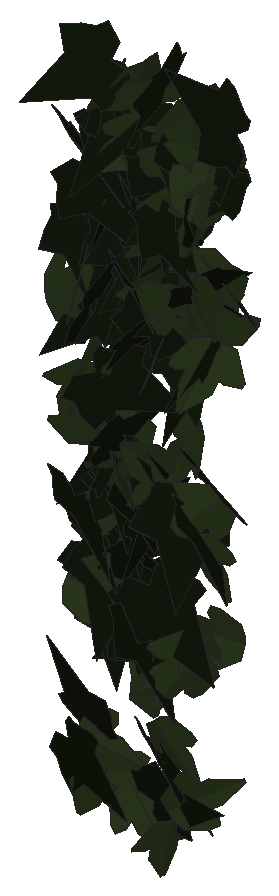
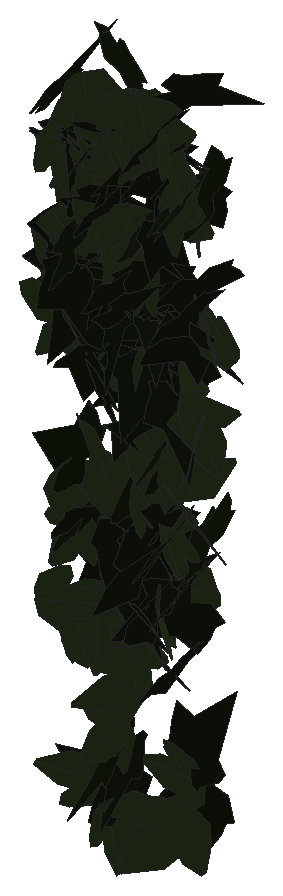
# SketchUp Ruby script. Lengths in inches.
U = 1.inch
M = Sketchup.active_model
def pt(a) = Geom::Point3d.new(a.map { |v| v * U })
def face(e, loops, mat)
  f = e.add_face(loops[0].map { |a| pt(a) })
  loops[1..].each { |l| e.add_face(l.map { |a| pt(a) }).erase! }
  f.material = f.back_material = mat if mat
  f
end
# faces: each face lists its corners as indices into pts; further lists are holes
def faces(e, pts, list, mat = nil) = list.each { |f| face(e, (f[0].is_a?(Array) ? f : [f]).map { |l| l.map { |i| pts[i] } }, mat) }
# xy, xz, yz: faces in a plane at the given z, y or x. An outline is a flat list of corners, or four numbers for a rectangle; further outlines are holes
def ring(l) = l.size == 4 ? [[l[0], l[1]], [l[2], l[1]], [l[2], l[3]], [l[0], l[3]]] : l.each_slice(2).to_a
def flat(e, list, mat, &to3) = list.each { |f| face(e, (f[0].is_a?(Array) ? f : [f]).map { |l| ring(l).map { |u, v| to3.(u, v) } }, mat) }
def xy(e, z, list, mat = nil) = flat(e, list, mat) { |x, y| [x, y, z] }
def xz(e, y, list, mat = nil) = flat(e, list, mat) { |x, z| [x, y, z] }
def yz(e, x, list, mat = nil) = flat(e, list, mat) { |y, z| [x, y, z] }
def lines(e, pts, list) = list.each { |a, b| e.add_line(pt(pts[a]), pt(pts[b])) }
# prism: a flat outline (further loops are holes) pulled along v
def prism(e, loops, v, mat = nil)
  f = face(e, loops, mat); d = Geom::Vector3d.new(v.map { |x| x * U })
  f.pushpull(f.normal.samedirection?(d) ? d.length : -d.length)
end
def box(e, o, s, mat = nil) = prism(e, [[o, [o[0] + s[0], o[1], o[2]], [o[0] + s[0], o[1] + s[1], o[2]], [o[0], o[1] + s[1], o[2]]]], [0, 0, s[2]], mat)
def at(x, y, z, deg = 0) = Geom::Transformation.translation(pt([x, y, z])) * Geom::Transformation.rotation(ORIGIN, Z_AXIS, deg.degrees)
def axes(o, x, y, z) = Geom::Transformation.new([*x, 0, *y, 0, *z, 0, *pt(o).to_a, 1])
def part(name) = M.definitions.add(name)
# library, detail: a bought-in or finely detailed component or shape, given as its bounding box
def library(name, o, s) = part(name).tap { |d| box(d.entities, o, s) }
def detail(e, o, s) = box(e.add_group.entities, o, s)
def put(e, d, t, mat = nil) = e.add_instance(d, t).tap { |i| i.material = mat if mat }
def group(e, t, mat = nil) = e.add_group.tap { |g| g.transformation = t; g.material = mat if mat }.entities
root = M.entities
M.materials.add("efeu1").color = [18, 25, 13]
M.materials.add("efeu2").color = [43, 57, 29]
c1 = part("ivyleaf_10")
p = [[0,0.5,-0.03],[-0.0625,2.02,-0.43],[-0.19,2.01,-0.46],[-0.54,1.05,-0.29],[-0.52,0.625,-0.18],[-0.83,0.76,-0.28],
  [-1.16,0.64,-0.33],[-1.15,0.33,-0.24],[-0.77,-0.39,0.02],[-0.3,-0.51,0.16],[0.04,-0.48,0.23],[-0.02,2.01,-0.4375],
  [-0.06,2.01,-0.43],[0.04,-0.49,0.23],[0.67,-0.49,0.14],[1.38,0.36,-0.2],[1.375,0.51,-0.24],[0.81,0.65,-0.19],
  [0.62,0.59,-0.15],[0.6,1.09,-0.28],[0.5,1.23,-0.31]]
faces(c1.entities,p,[[0,1,2,3,4,5,6,7,8,9,10],[11,12,0,13,14,15,16,17,18,19,20]],"efeu2")
c2 = part("ivyleaf_9")
p = [[1.54,2.16,1.25],[1.36,2.04,1.19],[-0.21,0.99,0.68],[-0.71,1.11,0.82],[-0.85,0.86,0.67],[-0.8,0.17,0.21],
  [-0.9,-0.01,0.1],[-0.67,-0.16,-0.02],[-0.08,-0.08,-0.05],[-0.03,-0.6,-0.4],[0.65,-0.88,-0.66],[0.83,-0.6,-0.49],
  [1.29,-0.42,-0.43],[1.8125,-0.07,-0.26],[1.21,0.44,0.15]]
faces(c2.entities,p,[[0,1,2,3,4,5,6,7,8,9,10,11,12,13,14]],"efeu1")
put(root,c1,axes([538.125,133.94,196.47],[-0.39679,-0.64724,0.32465],[-0.18478,-0.26744,-0.75901],[0.70012,-0.4374,-0.01633]))
put(root,c1,axes([538.48,134.31,202.8],[0.11635,0.17729,-0.84393],[-0.75483,0.43271,-0.01316],[0.41698,0.73384,0.21165]))
put(root,c1,axes([537.35,133.61,198.76],[0.54882,-0.22672,-0.62542],[0.56928,-0.25944,0.59361],[-0.3442,-0.7906,-0.01544]))
put(root,c2,axes([537.7,135.02,200.15],[-0.06376,-0.80231,0.12393],[-0.00926,-0.12358,-0.80484],[0.81178,-0.06443,0.00055]))
put(root,c1,axes([537.86,133.92,199.76],[0.55544,-0.65414,0.12328],[0.08516,-0.08941,-0.85812],[0.66019,0.56189,0.00697]))
put(root,c2,axes([537.78,134.2,200.82],[-0.09395,-0.79589,-0.21894],[0.03485,0.21634,-0.80136],[0.82472,-0.0998,0.00892]))
put(root,c2,axes([537.42,134.14,203.42],[0.58741,-0.58266,0.31966],[0.22728,-0.22478,-0.82737],[0.62451,0.62984,0.00043]))
put(root,c2,axes([538.35,133.75,186.3125],[0.41543,-0.40758,0.66623],[-0.47527,0.46689,0.58198],[-0.61976,-0.63124,0.00028]))
put(root,c1,axes([538.19,133.99,203.29],[0.50827,-0.5984,-0.32039],[-0.1439,0.29617,-0.78144],[0.66334,0.52275,0.07598]))
put(root,c1,axes([538.22,133.96,195.16],[-0.37011,0.76913,-0.02259],[-0.02989,0.01068,0.85325],[0.76888,0.37064,0.02229]))
put(root,c1,axes([538.09,134.36,197.58],[-0.22239,0.34672,-0.67417],[-0.01153,-0.70404,-0.35828],[-0.75801,-0.09102,0.20324]))
put(root,c2,axes([537.76,134.75,203.42],[0.47419,-0.67063,-0.05659],[0.01118,0.07706,-0.8196],[0.67292,0.4713,0.05349]))
put(root,c1,axes([538.29,134.74,204.97],[0.18494,-0.82253,0.03934],[0.01737,-0.03641,-0.84302],[0.82329,0.18553,0.00895]))
put(root,c2,axes([538.625,134.12,194.17],[-0.70422,0.30749,-0.05921],[0.05562,-0.02059,-0.76841],[-0.30816,-0.7064,-0.00337]))
put(root,c2,axes([538.68,133.97,205.98],[-0.66134,-0.30761,0.44171],[-0.35877,-0.26973,-0.72501],[0.40127,-0.74815,0.07978]))
put(root,c1,axes([538.23,134.01,194.68],[-0.74503,-0.50115,0.12123],[0.10127,0.06665,0.8979],[-0.50556,0.75188,0.00122]))
put(root,c2,axes([537.8,133.77,192.81],[0.42266,-0.77344,0.38973],[0.22896,-0.31845,-0.88029],[0.83527,0.47867,0.04409]))
put(root,c2,axes([538.81,133.8125,199.04],[-0.83451,0.00371,0.04795],[-0.04795,0.00106,-0.83451],[-0.00377,-0.83588,-0.00085]))
put(root,c2,axes([538.13,134.6875,191.55],[0.06127,-0.74917,0.31351],[0.01739,-0.31312,-0.75163],[0.81193,0.06324,-0.00756]))
put(root,c2,axes([538.75,133.83,196.84],[-0.1433,0.76912,-0.04322],[0.00941,-0.04221,-0.78235],[-0.77028,-0.1436,-0.00152]))
put(root,c2,axes([538.65,133.17,198.97],[-0.20834,0.44217,-0.79802],[-0.44743,0.66384,0.48464],[0.79508,0.48944,0.06362]))
put(root,c2,axes([537.89,133.46,185.6],[-0.00066,0.00453,-0.90717],[0.85758,0.29587,0.00085],[0.29587,-0.85757,-0.0045]))
put(root,c2,axes([538.29,134.65,189.38],[0.10566,-0.80781,0.08287],[0.01503,-0.08161,-0.81468],[0.81191,0.10663,0.0043]))
put(root,c2,axes([538.1,134.2,191.24],[0.03261,-0.15185,-0.83319],[0.40483,0.73517,-0.11815],[0.74389,-0.39343,0.10081]))
put(root,c1,axes([538.59,134.36,193.08],[0.75086,-0.1518,-0.07309],[-0.0714,0.01567,-0.76605],[0.1526,0.75425,0.0012]))
put(root,c2,axes([538.31,135.02,193.11],[0.16744,-0.77195,0.31509],[0.09835,-0.30085,-0.78933],[0.82796,0.19185,0.03004]))
put(root,c2,axes([538.17,133.66,192.39],[0.43223,-0.67212,0.32669],[0.17237,-0.27755,-0.79909],[0.72715,0.46531,-0.00477]))
put(root,c2,axes([538.82,134.6,202.29],[-0.39025,0.41969,-0.60601],[0.40578,-0.45015,-0.57306],[-0.61541,-0.56295,0.00644]))
put(root,c1,axes([538.52,134.7,191.02],[0.42529,-0.56538,0.53829],[0.36777,-0.39559,-0.70607],[0.68859,0.56048,0.04465]))
put(root,c1,axes([538.41,134.07,184.56],[-0.56636,-0.35628,-0.73053],[0.63915,0.35482,-0.66856],[0.5021,-0.85355,0.02701]))
put(root,c2,axes([538.65,134.82,204.08],[0.03151,-0.83531,-0.00958],[0.00016,0.00959,-0.8359],[0.83537,0.0315,0.00052]))
put(root,c1,axes([539.18,133.84,193.42],[-0.85254,0.32496,-0.16501],[-0.16092,0.041,0.91218],[0.327,0.86739,0.0187]))
put(root,c1,axes([539.34,134.13,195.35],[-0.4903,-0.3673,0.47625],[-0.29142,-0.39241,-0.60266],[0.52611,-0.55966,0.11001]))
put(root,c2,axes([538.74,134.9375,204.88],[0.08119,-0.8197,0.15461],[-0.00481,-0.15579,-0.82348],[0.83414,0.07889,-0.0198]))
put(root,c1,axes([538.4,133.77,185.78],[-0.09107,-0.04313,-0.87343],[0.82011,-0.30906,-0.07025],[-0.30358,-0.82198,0.07224]))
put(root,c2,axes([538.75,134.41,193.63],[0.08448,-0.46343,-0.66386],[0.03174,0.66885,-0.46288],[0.80899,0.02216,0.08749]))
put(root,c2,axes([539.19,134,204.42],[-0.77309,-0.18213,-0.23459],[0.27024,-0.16004,-0.76631],[0.12319,-0.79189,0.20882]))
put(root,c1,axes([539.18,134.7,205.51],[-0.09843,-0.84393,-0.00061],[0.00258,0.00031,-0.84964],[0.84392,-0.09843,0.00252]))
put(root,c2,axes([538.72,133.39,202.96],[-0.21372,-0.39699,-0.75706],[0.36359,0.66404,-0.45085],[0.77365,-0.42174,0.00275]))
put(root,c1,axes([539.08,134.82,194.43],[0.13144,-0.711,0.4615],[0.16516,-0.43658,-0.71965],[0.8314,0.19914,0.07]))
put(root,c2,axes([538.74,135.12,202.21],[0.10311,-0.68691,0.42719],[0.20691,-0.39393,-0.68336],[0.78201,0.1948,0.12448]))
put(root,c2,axes([538.92,134.51,200.82],[-0.30169,-0.59253,-0.4913],[0.24506,0.42629,-0.66461],[0.72967,-0.38816,0.02008]))
put(root,c2,axes([538.78,134.47,195.58],[0.41385,-0.68545,0.07201],[0.05112,-0.05324,-0.80053],[0.68732,0.41668,0.01618]))
put(root,c2,axes([538.95,133.87,191.16],[-0.03343,-0.93443,0.2435],[-0.0278,-0.24261,-0.93485],[0.96524,-0.03935,-0.01849]))
put(root,c1,axes([538.73,132.88,190.87],[0.15765,0.17631,0.79245],[0.5788,0.54163,-0.23565],[-0.56925,0.59955,-0.02015]))
put(root,c2,axes([539.74,133.74,198.74],[-0.15746,0.63778,0.51889],[-0.17108,0.49135,-0.65583],[-0.8042,-0.2294,0.03792]))
put(root,c2,axes([539.39,134.75,190.82],[-0.68632,0.01807,-0.40688],[0.40667,-0.01322,-0.68656],[-0.02229,-0.79775,0.00216]))
put(root,c2,axes([538.68,134.85,190.97],[0.33065,-0.32867,0.68533],[0.52789,-0.43841,-0.46494],[0.54685,0.62194,0.03443]))
put(root,c1,axes([539.74,134.18,204.11],[0.3884,0.38225,-0.66317],[-0.58372,-0.33316,-0.5339],[-0.49516,0.69257,0.10919]))
put(root,c2,axes([539.63,135.22,199.79],[-0.48758,-0.49086,0.40875],[-0.20865,-0.36362,-0.68556],[0.60372,-0.5221,0.09317]))
put(root,c2,axes([539.26,133.14,195.12],[0.04861,0.6858,-0.38367],[-0.05895,0.3865,0.6834],[0.78361,-0.01347,0.07521]))
put(root,c2,axes([539.47,133.83,192.05],[-0.06765,0.11804,-0.82061],[-0.25856,0.77927,0.13341],[0.7877,0.26592,-0.02669]))
put(root,c1,axes([539.43,134.4,200.57],[-0.73866,0.29447,-0.24979],[0.22395,-0.11254,-0.79493],[-0.31457,-0.77159,0.02061]))
put(root,c2,axes([539.7,133.91,197.63],[0.1711,0.75323,0.1979],[0.04561,0.19258,-0.77241],[-0.77745,0.17707,-0.00175]))
put(root,c1,axes([539.68,133.83,197.64],[0.01621,-0.75073,0.26481],[0.05305,-0.26326,-0.74957],[0.79429,0.0329,0.04466]))
put(root,c1,axes([539.75,134.35,205.33],[-0.53255,-0.62878,-0.11069],[0.05267,0.10039,-0.82363],[0.63627,-0.53459,-0.02447]))
put(root,c2,axes([539.45,134.22,192.77],[0.64452,-0.55319,-0.25391],[0.19238,-0.16572,0.84937],[-0.57748,-0.67262,-0.00044]))
put(root,c1,axes([539.66,134.5,189.28],[0.52893,0.56042,-0.0564],[-0.03982,-0.03997,-0.77061],[-0.56185,0.53043,0.00153]))
put(root,c2,axes([539.38,132.79,197.42],[0.08838,-0.02853,-0.91244],[0.18508,0.89822,-0.01016],[0.89392,-0.18315,0.09231]))
put(root,c2,axes([540.35,133.875,189.58],[-0.68311,0.31373,0.19461],[-0.18307,0.06757,-0.75157],[-0.3206,-0.70707,0.01452]))
put(root,c2,axes([540.19,134.92,199.65],[-0.29134,-0.85831,-0.02374],[0.02449,-0.03337,0.90577],[-0.85829,0.29039,0.03391]))
put(root,c1,axes([539.87,134.37,201.9],[-0.30237,-0.66513,-0.40057],[0.17699,0.35951,-0.73055],[0.756,-0.35019,0.01082]))
put(root,c2,axes([539.3,134.66,194.21],[0.65805,-0.06727,-0.51152],[0.50623,-0.07573,0.66121],[-0.09952,-0.83003,-0.01888]))
put(root,c1,axes([540.23,134.7,193.93],[-0.38247,-0.4744,-0.72554],[-0.44713,-0.57142,0.60934],[-0.74265,0.58836,0.00679]))
put(root,c2,axes([540.06,134.72,193.16],[-0.34013,0.42247,-0.77528],[0.47469,-0.61303,-0.54231],[-0.74445,-0.58391,0.00842]))
put(root,c1,axes([539.77,133.85,184.52],[0.40929,0.63903,0.34305],[0.18398,0.28954,-0.75886],[-0.70156,0.44873,0.00112]))
put(root,c2,axes([540.37,133.5,198.86],[-0.31113,0.5612,-0.46962],[0.10165,-0.47222,-0.63165],[-0.72468,-0.30718,0.11302]))
put(root,c2,axes([539.77,133.71,199.41],[-0.20769,-0.1469,0.7938],[0.31409,-0.76977,-0.06027],[0.74367,0.28409,0.24715]))
put(root,c2,axes([540.44,134.26,200.13],[-0.77869,-0.3229,0.02286],[-0.01891,-0.01406,-0.84297],[0.32316,-0.7789,0.00574]))
put(root,c2,axes([540.4375,134.2,199.34],[0.49129,0.07557,-0.68058],[-0.68457,0.07407,-0.48594],[0.01624,0.8361,0.10457]))
put(root,c2,axes([539.91,134.34,203.52],[0.32212,-0.68183,-0.35126],[-0.0747,0.35128,-0.75038],[0.76335,0.3221,0.07479]))
put(root,c2,axes([540.25,133.82,186.27],[0.70306,-0.07472,-0.51763],[-0.51061,0.08956,-0.70646],[0.11314,0.86846,0.02832]))
put(root,c1,axes([540.04,133.88,188.31],[0.09913,-0.15937,-0.9898],[0.4558,0.89306,-0.09814],[0.89295,-0.43817,0.15998]))
put(root,c2,axes([540.15,135.01,201.21],[-0.30566,-0.62853,0.46493],[0.08178,-0.52217,-0.65214],[0.77751,-0.19218,0.25137]))
put(root,c1,axes([540.07,134.31,197.25],[0.09029,-0.75813,-0.35778],[0.19632,-0.33072,0.75033],[-0.815,-0.16365,0.14111]))
put(root,c1,axes([540.52,134.11,201.53],[-0.28569,-0.77837,-0.12874],[0.04539,0.12048,-0.82914],[0.78764,-0.28927,0.00108]))
put(root,c1,axes([539.99,133.95,203.82],[-0.42246,-0.11546,-0.7096],[0.69521,0.14407,-0.43734],[0.18316,-0.81318,0.02327]))
put(root,c2,axes([540.98,133.45,206.21],[-0.4704,0.69738,0.26632],[-0.13378,0.23093,-0.84102],[-0.73441,-0.48875,-0.01738]))
put(root,c2,axes([540.05,133.58,189.91],[0.45399,-0.8519,-0.09464],[-0.04375,0.08393,-0.96532],[0.85602,0.4561,0.00085]))
put(root,c1,axes([540.67,133.67,201.06],[0.09603,-0.80694,-0.22992],[-0.03691,0.22713,-0.81258],[0.83824,0.10245,-0.00944]))
put(root,c2,axes([540.37,134.79,202.4],[-0.05756,-0.81263,0.14807],[-0.028,-0.14642,-0.81448],[0.82553,-0.06163,-0.0173]))
put(root,c2,axes([540.96,134.89,202.5],[-0.67322,-0.40069,0.27581],[-0.15953,-0.26301,-0.77151],[0.45954,-0.67832,0.13622]))
put(root,c1,axes([540.95,133.44,200.05],[-0.72374,-0.41631,0.13122],[-0.10528,-0.0801,-0.83477],[0.42362,-0.73116,0.01674]))
put(root,c1,axes([540.85,133.83,183.875],[-0.19516,-0.74584,0.00108],[0.00212,-0.00167,-0.77095],[0.74584,-0.19516,0.00247]))
put(root,c2,axes([540.54,134.77,198.04],[-0.18715,-0.69432,-0.37775],[0.15437,0.34862,-0.71724],[0.77521,-0.23704,0.05163]))
put(root,c2,axes([540.67,134.61,204.54],[-0.35037,-0.70614,-0.2528],[0.241,0.15824,-0.77601],[0.71026,-0.40203,0.1386]))
put(root,c1,axes([541.03,134.3,202.6],[-0.2766,-0.71406,0.32298],[-0.04181,-0.32857,-0.76224],[0.7826,-0.26993,0.07343]))
put(root,c2,axes([540.96,134.71,197.39],[-0.68543,0.07223,-0.39946],[0.40032,-0.00967,-0.68866],[-0.06729,-0.79327,-0.02798]))
put(root,c1,axes([541.01,134.64,195.36],[0.68633,-0.48896,-0.21172],[-0.16529,0.13283,-0.84261],[0.50654,0.70585,0.0119]))
put(root,c1,axes([540.61,134,186.62],[-0.61672,0.19329,-0.48174],[0.46398,-0.13013,-0.6462],[-0.23272,-0.77168,-0.01169]))
put(root,c1,axes([540.79,133.88,203.9375],[-0.71203,-0.2036,-0.34563],[0.34219,0.05915,-0.73979],[0.20932,-0.78927,0.03372]))
put(root,c1,axes([540.97,134.12,199.53],[-0.64368,0.46513,-0.12795],[0.09788,-0.08298,-0.79409],[-0.47237,-0.65101,0.00981]))
put(root,c1,axes([541.37,134,190.12],[-0.89778,0.06043,0.2919],[-0.29146,0.01631,-0.8998],[-0.06251,-0.9439,0.00314]))
put(root,c2,axes([540.81,133.78,185.98],[0.71751,-0.37346,-0.34054],[-0.30149,0.15835,-0.80889],[0.40564,0.77828,0.00117]))
put(root,c1,axes([541.2,134.51,205.4],[-0.24977,-0.79687,-0.10201],[0.01042,0.1036,-0.83484],[0.80331,-0.24911,-0.02089]))
put(root,c2,axes([540.62,133.49,198.78],[-0.14591,-0.00995,0.93928],[0.9231,0.17443,0.14524],[-0.17388,0.93441,-0.01711]))
put(root,c2,axes([540.44,133.88,184.54],[0.26024,-0.17699,0.81736],[0.68667,-0.44341,-0.31464],[0.47738,0.7343,0.00701]))
put(root,c2,axes([540.57,133.51,191.05],[-0.18218,-0.3779,-0.92751],[0.69691,0.62923,-0.39325],[0.7193,-0.70536,0.1461]))
put(root,c2,axes([540.96,134.49,193.2],[-0.21972,-0.92359,-0.06457],[0.01902,0.06185,-0.94935],[0.92565,-0.2205,0.00417]))
put(root,c1,axes([541.29,134.46,204.74],[-0.58674,-0.60124,-0.00818],[0.00453,0.00701,-0.84008],[0.60127,-0.58675,-0.00166]))
put(root,c2,axes([541.45,134.41,199.96],[0.06774,0.75149,-0.39845],[-0.03012,-0.39734,-0.75452],[-0.85005,0.07396,-0.00501]))
put(root,c2,axes([540.9,134.49,203.9],[0.19144,-0.80566,0.1529],[0.0174,-0.15299,-0.8279],[0.81986,0.19137,-0.01814]))
put(root,c2,axes([540.98,133.35,202.45],[0.33976,-0.66029,-0.33286],[-0.08623,0.32843,-0.73953],[0.7344,0.34404,0.06716]))
put(root,c1,axes([541.8125,133.76,189.14],[-0.24611,-0.34737,0.74132],[-0.46101,-0.58088,-0.42524],[0.67653,-0.52221,-0.0201]))
put(root,c2,axes([541.25,134.28,199.59],[0.69987,0.37017,-0.14344],[-0.12914,-0.06263,-0.79172],[-0.3754,0.71166,0.00493]))
put(root,c1,axes([541.85,134.4,193.63],[-0.44954,-0.26961,0.57998],[-0.4063,-0.42711,-0.51347],[0.49395,-0.59669,0.10548]))
put(root,c1,axes([541.7,133.88,189.51],[-0.28712,-0.7048,0.55914],[-0.10999,-0.55502,-0.7561],[0.89291,-0.29501,0.08666]))
put(root,c2,axes([541.7,133.96,202.04],[0.03686,-0.37409,0.75682],[0.25884,0.72606,0.34628],[-0.80356,0.21672,0.14626]))
put(root,c2,axes([541.88,134.31,198.5],[-0.66942,0.28651,-0.3096],[0.2615,-0.17384,-0.72627],[-0.331,-0.71677,0.05238]))
put(root,c2,axes([542.16,134.73,203.8125],[-0.80924,-0.03063,0.18632],[-0.18629,-0.00429,-0.80981],[0.03081,-0.8304,-0.00269]))
put(root,c1,axes([541.85,134.72,203.85],[-0.2909,-0.77456,0.09112],[-0.03437,-0.08443,-0.82738],[0.77914,-0.29292,-0.00248]))
put(root,c1,axes([541.39,133.82,184.74],[-0.14534,-0.34891,0.74435],[0.37081,0.6468,0.37558],[-0.73368,0.39601,0.04237]))
put(root,c1,axes([541.86,134.32,198.15],[0.52842,0.51896,-0.39533],[-0.30524,-0.25295,-0.74005],[-0.57657,0.60954,0.02947]))
put(root,c1,axes([541.88,134.18,202.88],[-0.08965,-0.77778,0.38312],[0.04112,-0.38854,-0.77916],[0.86604,-0.06207,0.07666]))
put(root,c1,axes([541.625,134.3,192.38],[-0.69589,0.12671,-0.34042],[0.32555,-0.10874,-0.70597],[-0.16111,-0.76702,0.04385]))
put(root,c1,axes([542.28,134.22,200.88],[-0.5557,-0.327,0.56889],[-0.45954,-0.33821,-0.64328],[0.4684,-0.71976,0.04381]))
put(root,c1,axes([541.87,133.67,202.99],[0.23474,0.64527,-0.63514],[0.10199,0.63312,0.68091],[0.89966,-0.24014,0.08853]))
put(root,c1,axes([542.48,134.32,189.91],[-0.08914,0.00393,-0.79023],[-0.78997,0.02042,0.08921],[0.02073,0.79498,0.00162]))
put(root,c2,axes([541.35,134.43,192.89],[0.36982,-0.73572,0.38608],[0.20812,-0.3271,-0.82267],[0.80438,0.42288,0.03535]))
put(root,c2,axes([542.26,134.62,203.625],[-0.82125,-0.03334,-0.01598],[0.01622,-0.0054,-0.82191],[0.03323,-0.82139,0.00605]))
put(root,c1,axes([541.94,134.48,198.82],[-0.66399,-0.63073,0.06055],[0.04857,0.03678,0.91578],[-0.63176,0.66573,0.00677]))
put(root,c2,axes([541.38,134.41,194.48],[0.4126,-0.46789,0.54841],[0.40733,-0.37002,-0.62216],[0.59477,0.57799,0.04565]))
put(root,c2,axes([541.47,134.74,200.69],[0.53974,-0.51827,0.31041],[0.23164,-0.2069,-0.74821],[0.55795,0.58725,0.01034]))
put(root,c2,axes([542.31,134.68,204.83],[-0.01018,-0.94154,0.03423],[0.00669,0.03416,0.94158],[-0.94214,0.01042,0.00631]))
put(root,c2,axes([542,133.56,200.64],[0.43978,0.67539,0.11118],[0.05404,0.09748,-0.80591],[-0.68234,0.44302,0.00783]))
put(root,c1,axes([542.02,133.49,200.73],[-0.74029,0.26566,-0.16374],[0.14956,-0.06793,-0.7864],[-0.2739,-0.75513,0.01314]))
